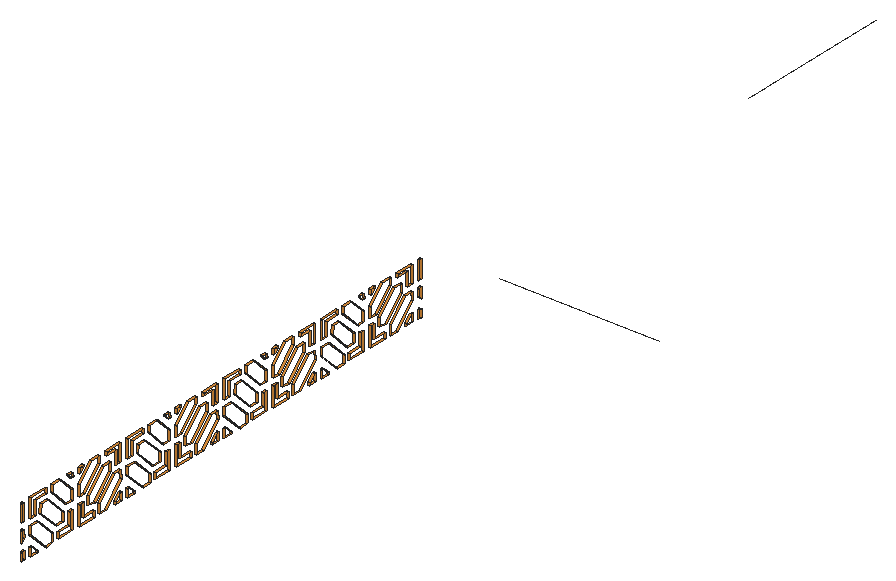
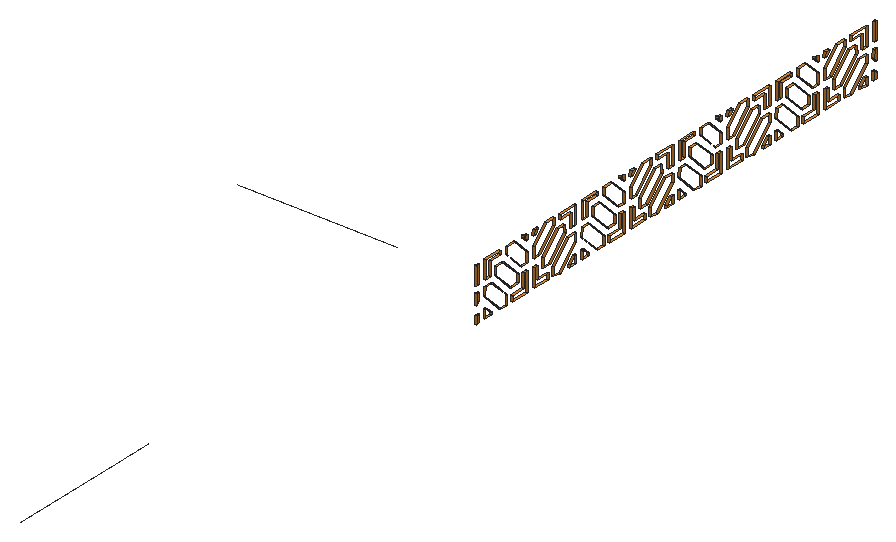
# SketchUp Ruby script. Lengths in inches.
U = 1.inch
M = Sketchup.active_model
def pt(a) = Geom::Point3d.new(a.map { |v| v * U })
def face(e, loops, mat)
  f = e.add_face(loops[0].map { |a| pt(a) })
  loops[1..].each { |l| e.add_face(l.map { |a| pt(a) }).erase! }
  f.material = f.back_material = mat if mat
  f
end
# faces: each face lists its corners as indices into pts; further lists are holes
def faces(e, pts, list, mat = nil) = list.each { |f| face(e, (f[0].is_a?(Array) ? f : [f]).map { |l| l.map { |i| pts[i] } }, mat) }
# xy, xz, yz: faces in a plane at the given z, y or x. An outline is a flat list of corners, or four numbers for a rectangle; further outlines are holes
def ring(l) = l.size == 4 ? [[l[0], l[1]], [l[2], l[1]], [l[2], l[3]], [l[0], l[3]]] : l.each_slice(2).to_a
def flat(e, list, mat, &to3) = list.each { |f| face(e, (f[0].is_a?(Array) ? f : [f]).map { |l| ring(l).map { |u, v| to3.(u, v) } }, mat) }
def xy(e, z, list, mat = nil) = flat(e, list, mat) { |x, y| [x, y, z] }
def xz(e, y, list, mat = nil) = flat(e, list, mat) { |x, z| [x, y, z] }
def yz(e, x, list, mat = nil) = flat(e, list, mat) { |y, z| [x, y, z] }
def lines(e, pts, list) = list.each { |a, b| e.add_line(pt(pts[a]), pt(pts[b])) }
# prism: a flat outline (further loops are holes) pulled along v
def prism(e, loops, v, mat = nil)
  f = face(e, loops, mat); d = Geom::Vector3d.new(v.map { |x| x * U })
  f.pushpull(f.normal.samedirection?(d) ? d.length : -d.length)
end
def box(e, o, s, mat = nil) = prism(e, [[o, [o[0] + s[0], o[1], o[2]], [o[0] + s[0], o[1] + s[1], o[2]], [o[0], o[1] + s[1], o[2]]]], [0, 0, s[2]], mat)
def at(x, y, z, deg = 0) = Geom::Transformation.translation(pt([x, y, z])) * Geom::Transformation.rotation(ORIGIN, Z_AXIS, deg.degrees)
def axes(o, x, y, z) = Geom::Transformation.new([*x, 0, *y, 0, *z, 0, *pt(o).to_a, 1])
def part(name) = M.definitions.add(name)
# library, detail: a bought-in or finely detailed component or shape, given as its bounding box
def library(name, o, s) = part(name).tap { |d| box(d.entities, o, s) }
def detail(e, o, s) = box(e.add_group.entities, o, s)
def put(e, d, t, mat = nil) = e.add_instance(d, t).tap { |i| i.material = mat if mat }
def group(e, t, mat = nil) = e.add_group.tap { |g| g.transformation = t; g.material = mat if mat }.entities
root = M.entities
M.materials.add("1056 AP 9903 Mellow Melon-N").color = [219, 142, 59]
xy(root,193.38,[[14.35,18.88,15.0625,21.91],[14.35,64.22,15.0625,67.26],[14.35,109.57,15.0625,112.6],[14.35,154.91,15.0625,157.94],[14.35,200.25,15.0625,201.3125]],"1056 AP 9903 Mellow Melon-N")
xy(root,193.61,[[14.35,14.79,15.0625,16.07],[14.35,41.65,15.0625,48.53],[14.35,51.11,15.0625,54.08],[14.35,58.41,15.0625,61.42],[14.35,87,15.0625,93.87],
  [14.35,96.45,15.0625,99.42],[14.35,103.75,15.0625,106.76],[14.35,132.34,15.0625,139.21],[14.35,141.79,15.0625,144.77],[14.35,149.1,15.0625,152.1],
  [14.35,177.68,15.0625,184.56],[14.35,187.14,15.0625,190.11],[14.35,194.44,15.0625,197.45]],"1056 AP 9903 Mellow Melon-N")
xy(root,193.8125,[[14.35,31.88,15.0625,38.38],[14.35,77.22,15.0625,83.72],[14.35,122.57,15.0625,129.07],[14.35,167.91,15.0625,174.41]],"1056 AP 9903 Mellow Melon-N")
xy(root,195.78,[[14.35,43.37,15.0625,48.53],[14.35,88.72,15.0625,93.87],[14.35,134.06,15.0625,139.21],[14.35,179.4,15.0625,184.56]],"1056 AP 9903 Mellow Melon-N")
xy(root,195.96,[[14.35,31.88,15.0625,37.08],[14.35,77.22,15.0625,82.42],[14.35,122.57,15.0625,127.77],[14.35,167.91,15.0625,173.11]],"1056 AP 9903 Mellow Melon-N")
xy(root,196.39,[[14.35,18.88,15.0625,19.75],[14.35,64.22,15.0625,65.1],[14.35,109.57,15.0625,110.44],[14.35,154.91,15.0625,155.79],[14.35,200.25,15.0625,201.13]],"1056 AP 9903 Mellow Melon-N")
xy(root,196.64,[[14.35,15.22,15.0625,16.07],[14.35,60.57,15.0625,61.42],[14.35,105.91,15.0625,106.76],[14.35,151.25,15.0625,152.1],[14.35,196.6,15.0625,197.45]],"1056 AP 9903 Mellow Melon-N")
xy(root,198.54,[[14.35,30.98,15.0625,34.05],[14.35,76.32,15.0625,79.39],[14.35,121.67,15.0625,124.73],[14.35,167.01,15.0625,170.08]],"1056 AP 9903 Mellow Melon-N")
xy(root,200.6875,[[14.35,37.08,15.0625,38.38],[14.35,82.42,15.0625,83.72],[14.35,127.77,15.0625,129.07],[14.35,173.11,15.0625,174.41]],"1056 AP 9903 Mellow Melon-N")
xy(root,200.98,[[14.35,41.65,15.0625,43.37],[14.35,87,15.0625,88.72],[14.35,132.34,15.0625,134.06],[14.35,177.68,15.0625,179.4]],"1056 AP 9903 Mellow Melon-N")
xy(root,203.58,[[14.35,41.65,15.0625,44.2],[14.35,87,15.0625,89.54],[14.35,132.34,15.0625,134.89],[14.35,177.68,15.0625,180.23]],"1056 AP 9903 Mellow Melon-N")
xy(root,203.69,[[14.35,18.88,15.0625,22.375],[14.35,35.75,15.0625,38.38],[14.35,64.22,15.0625,67.72],[14.35,81.09,15.0625,83.72],[14.35,109.57,15.0625,113.0625],
  [14.35,126.4375,15.0625,129.07],[14.35,154.91,15.0625,158.41],[14.35,171.78,15.0625,174.41],[14.35,200.25,15.0625,201.3125]],"1056 AP 9903 Mellow Melon-N")
xy(root,204.01,[[14.35,14.79,15.0625,15.64],[14.35,58.01,15.0625,60.99],[14.35,103.35,15.0625,106.33],[14.35,148.7,15.0625,151.67],[14.35,194.04,15.0625,197.02]],"1056 AP 9903 Mellow Melon-N")
xy(root,206.27,[[14.35,18.88,15.0625,21.05],[14.35,64.22,15.0625,66.39],[14.35,109.57,15.0625,111.73],[14.35,154.91,15.0625,157.08],[14.35,200.25,15.0625,201.3125]],"1056 AP 9903 Mellow Melon-N")
xy(root,206.61,[[14.35,14.79,15.0625,15.64],[14.35,58.84,15.0625,60.99],[14.35,104.18,15.0625,106.33],[14.35,149.53,15.0625,151.67],[14.35,194.87,15.0625,197.02]],"1056 AP 9903 Mellow Melon-N")
xy(root,208.78,[[14.35,52.85,15.0625,56.26],[14.35,98.2,15.0625,101.6],[14.35,143.54,15.0625,146.95],[14.35,188.88,15.0625,192.29]],"1056 AP 9903 Mellow Melon-N")
xy(root,208.85,[[14.35,24.08,15.0625,27.14],[14.35,69.42,15.0625,72.49],[14.35,114.77,15.0625,117.83],[14.35,160.11,15.0625,163.17]],"1056 AP 9903 Mellow Melon-N")
xy(root,211.38,[[14.35,41.65,15.0625,42.08],[14.35,87,15.0625,87.42],[14.35,132.34,15.0625,132.76],[14.35,177.68,15.0625,178.11]],"1056 AP 9903 Mellow Melon-N")
xy(root,211.43,[[14.35,21.05,15.0625,26.25],[14.35,37.94,15.0625,38.8125],[14.35,66.39,15.0625,71.59],[14.35,83.29,15.0625,84.16],[14.35,111.73,15.0625,116.93],
  [14.35,128.63,15.0625,129.5],[14.35,157.08,15.0625,162.28],[14.35,173.97,15.0625,174.84]],"1056 AP 9903 Mellow Melon-N")
xy(root,211.8125,[[14.35,54.11,15.0625,58.84],[14.35,99.46,15.0625,104.18],[14.35,144.8,15.0625,149.53],[14.35,190.14,15.0625,194.87]],"1056 AP 9903 Mellow Melon-N")
xy(root,213.11,[[14.35,14.79,15.0625,15.64],[14.35,47.26,15.0625,51.11],[14.35,54.11,15.0625,60.99],[14.35,92.61,15.0625,96.45],[14.35,99.46,15.0625,106.33],
  [14.35,137.95,15.0625,141.79],[14.35,144.8,15.0625,151.67],[14.35,183.29,15.0625,187.14],[14.35,190.14,15.0625,197.02]],"1056 AP 9903 Mellow Melon-N")
xy(root,213.15,[[14.35,18.88,15.0625,26.25],[14.35,28.85,15.0625,32.77],[14.35,36.65,15.0625,38.38],[14.35,64.22,15.0625,71.59],[14.35,74.19,15.0625,78.11],
  [14.35,81.99,15.0625,83.72],[14.35,109.57,15.0625,116.93],[14.35,119.53,15.0625,123.46],[14.35,127.33,15.0625,129.07],[14.35,154.91,15.0625,162.28],
  [14.35,164.88,15.0625,168.8],[14.35,172.68,15.0625,174.41],[14.35,200.25,15.0625,201.3125]],"1056 AP 9903 Mellow Melon-N")
xz(root,14.79,[[14.35,193.61,15.0625,196.21],[14.35,199.66,15.0625,204.01],[14.35,206.61,15.0625,213.11]],"1056 AP 9903 Mellow Melon-N")
xz(root,15.64,[[14.35,206.61,15.0625,213.11]],"1056 AP 9903 Mellow Melon-N")
xz(root,16.07,[[14.35,193.61,15.0625,196.64]],"1056 AP 9903 Mellow Melon-N")
xz(root,18.88,[[14.35,193.38,15.0625,196.39],[14.35,200.72,15.0625,203.69],[14.35,206.27,15.0625,213.15]],"1056 AP 9903 Mellow Melon-N")
xz(root,21.05,[[14.35,206.27,15.0625,211.43]],"1056 AP 9903 Mellow Melon-N")
xz(root,21.91,[[14.35,193.38,15.0625,194.23]],"1056 AP 9903 Mellow Melon-N")
xz(root,26.25,[[14.35,211.43,15.0625,213.15]],"1056 AP 9903 Mellow Melon-N")
xz(root,28.85,[[14.35,210.6,15.0625,213.15]],"1056 AP 9903 Mellow Melon-N")
xz(root,29.28,[[14.35,193.8125,15.0625,196.79]],"1056 AP 9903 Mellow Melon-N")
xz(root,31.88,[[14.35,193.8125,15.0625,195.96]],"1056 AP 9903 Mellow Melon-N")
xz(root,34.05,[[14.35,198.54,15.0625,201.95]],"1056 AP 9903 Mellow Melon-N")
xz(root,36.65,[[14.35,212.72,15.0625,213.15]],"1056 AP 9903 Mellow Melon-N")
xz(root,37.08,[[14.35,195.96,15.0625,200.6875]],"1056 AP 9903 Mellow Melon-N")
xz(root,38.38,[[14.35,193.8125,15.0625,200.6875],[14.35,203.69,15.0625,207.54]],"1056 AP 9903 Mellow Melon-N")
xz(root,41.65,[[14.35,193.61,15.0625,200.98],[14.35,203.58,15.0625,207.5],[14.35,211.38,15.0625,213.11]],"1056 AP 9903 Mellow Melon-N")
xz(root,43.37,[[14.35,195.78,15.0625,200.98],[14.35,212.67,15.0625,213.55]],"1056 AP 9903 Mellow Melon-N")
xz(root,45.95,[[14.35,198.8125,15.0625,201.875]],"1056 AP 9903 Mellow Melon-N")
xz(root,48.53,[[14.35,193.61,15.0625,195.78]],"1056 AP 9903 Mellow Melon-N")
xz(root,51.11,[[14.35,193.61,15.0625,197.11],[14.35,210.48,15.0625,213.11]],"1056 AP 9903 Mellow Melon-N")
xz(root,54.11,[[14.35,211.8125,15.0625,213.11]],"1056 AP 9903 Mellow Melon-N")
xz(root,56.26,[[14.35,205.71,15.0625,208.78]],"1056 AP 9903 Mellow Melon-N")
xz(root,58.41,[[14.35,193.61,15.0625,194.49]],"1056 AP 9903 Mellow Melon-N")
xz(root,58.84,[[14.35,206.61,15.0625,211.8125]],"1056 AP 9903 Mellow Melon-N")
xz(root,60.99,[[14.35,206.61,15.0625,213.11]],"1056 AP 9903 Mellow Melon-N")
xz(root,61.42,[[14.35,193.61,15.0625,196.64]],"1056 AP 9903 Mellow Melon-N")
xz(root,64.22,[[14.35,193.38,15.0625,196.39],[14.35,200.72,15.0625,203.69],[14.35,206.27,15.0625,213.15]],"1056 AP 9903 Mellow Melon-N")
xz(root,66.39,[[14.35,206.27,15.0625,211.43]],"1056 AP 9903 Mellow Melon-N")
xz(root,67.26,[[14.35,193.38,15.0625,194.23]],"1056 AP 9903 Mellow Melon-N")
xz(root,71.59,[[14.35,211.43,15.0625,213.15]],"1056 AP 9903 Mellow Melon-N")
xz(root,74.19,[[14.35,210.6,15.0625,213.15]],"1056 AP 9903 Mellow Melon-N")
xz(root,74.625,[[14.35,193.8125,15.0625,196.79]],"1056 AP 9903 Mellow Melon-N")
xz(root,77.22,[[14.35,193.8125,15.0625,195.96]],"1056 AP 9903 Mellow Melon-N")
xz(root,79.39,[[14.35,198.54,15.0625,201.95]],"1056 AP 9903 Mellow Melon-N")
xz(root,81.99,[[14.35,212.72,15.0625,213.15]],"1056 AP 9903 Mellow Melon-N")
xz(root,82.42,[[14.35,195.96,15.0625,200.6875]],"1056 AP 9903 Mellow Melon-N")
xz(root,83.72,[[14.35,193.8125,15.0625,200.6875],[14.35,203.69,15.0625,207.54]],"1056 AP 9903 Mellow Melon-N")
xz(root,87,[[14.35,193.61,15.0625,200.98],[14.35,203.58,15.0625,207.5],[14.35,211.38,15.0625,213.11]],"1056 AP 9903 Mellow Melon-N")
xz(root,88.72,[[14.35,195.78,15.0625,200.98],[14.35,212.67,15.0625,213.55]],"1056 AP 9903 Mellow Melon-N")
xz(root,91.29,[[14.35,198.8125,15.0625,201.875]],"1056 AP 9903 Mellow Melon-N")
xz(root,93.87,[[14.35,193.61,15.0625,195.78]],"1056 AP 9903 Mellow Melon-N")
xz(root,96.45,[[14.35,193.61,15.0625,197.11],[14.35,210.48,15.0625,213.11]],"1056 AP 9903 Mellow Melon-N")
xz(root,99.46,[[14.35,211.8125,15.0625,213.11]],"1056 AP 9903 Mellow Melon-N")
xz(root,101.6,[[14.35,205.71,15.0625,208.78]],"1056 AP 9903 Mellow Melon-N")
xz(root,103.75,[[14.35,193.61,15.0625,194.49]],"1056 AP 9903 Mellow Melon-N")
xz(root,104.18,[[14.35,206.61,15.0625,211.8125]],"1056 AP 9903 Mellow Melon-N")
xz(root,106.33,[[14.35,206.61,15.0625,213.11]],"1056 AP 9903 Mellow Melon-N")
xz(root,106.76,[[14.35,193.61,15.0625,196.64]],"1056 AP 9903 Mellow Melon-N")
xz(root,109.57,[[14.35,193.38,15.0625,196.39],[14.35,200.72,15.0625,203.69],[14.35,206.27,15.0625,213.15]],"1056 AP 9903 Mellow Melon-N")
xz(root,111.73,[[14.35,206.27,15.0625,211.43]],"1056 AP 9903 Mellow Melon-N")
xz(root,112.6,[[14.35,193.38,15.0625,194.23]],"1056 AP 9903 Mellow Melon-N")
xz(root,116.93,[[14.35,211.43,15.0625,213.15]],"1056 AP 9903 Mellow Melon-N")
xz(root,119.53,[[14.35,210.6,15.0625,213.15]],"1056 AP 9903 Mellow Melon-N")
xz(root,119.97,[[14.35,193.8125,15.0625,196.79]],"1056 AP 9903 Mellow Melon-N")
xz(root,122.57,[[14.35,193.8125,15.0625,195.96]],"1056 AP 9903 Mellow Melon-N")
xz(root,124.73,[[14.35,198.54,15.0625,201.95]],"1056 AP 9903 Mellow Melon-N")
xz(root,127.33,[[14.35,212.72,15.0625,213.15]],"1056 AP 9903 Mellow Melon-N")
xz(root,127.77,[[14.35,195.96,15.0625,200.6875]],"1056 AP 9903 Mellow Melon-N")
xz(root,129.07,[[14.35,193.8125,15.0625,200.6875],[14.35,203.69,15.0625,207.54]],"1056 AP 9903 Mellow Melon-N")
xz(root,132.34,[[14.35,193.61,15.0625,200.98],[14.35,203.58,15.0625,207.5],[14.35,211.38,15.0625,213.11]],"1056 AP 9903 Mellow Melon-N")
xz(root,134.06,[[14.35,195.78,15.0625,200.98],[14.35,212.67,15.0625,213.55]],"1056 AP 9903 Mellow Melon-N")
xz(root,136.64,[[14.35,198.8125,15.0625,201.875]],"1056 AP 9903 Mellow Melon-N")
xz(root,139.21,[[14.35,193.61,15.0625,195.78]],"1056 AP 9903 Mellow Melon-N")
xz(root,141.79,[[14.35,193.61,15.0625,197.11],[14.35,210.48,15.0625,213.11]],"1056 AP 9903 Mellow Melon-N")
xz(root,144.8,[[14.35,211.8125,15.0625,213.11]],"1056 AP 9903 Mellow Melon-N")
xz(root,146.95,[[14.35,205.71,15.0625,208.78]],"1056 AP 9903 Mellow Melon-N")
xz(root,149.1,[[14.35,193.61,15.0625,194.49]],"1056 AP 9903 Mellow Melon-N")
xz(root,149.53,[[14.35,206.61,15.0625,211.8125]],"1056 AP 9903 Mellow Melon-N")
xz(root,151.67,[[14.35,206.61,15.0625,213.11]],"1056 AP 9903 Mellow Melon-N")
xz(root,152.1,[[14.35,193.61,15.0625,196.64]],"1056 AP 9903 Mellow Melon-N")
xz(root,154.91,[[14.35,193.38,15.0625,196.39],[14.35,200.72,15.0625,203.69],[14.35,206.27,15.0625,213.15]],"1056 AP 9903 Mellow Melon-N")
xz(root,157.08,[[14.35,206.27,15.0625,211.43]],"1056 AP 9903 Mellow Melon-N")
xz(root,157.94,[[14.35,193.38,15.0625,194.23]],"1056 AP 9903 Mellow Melon-N")
xz(root,162.28,[[14.35,211.43,15.0625,213.15]],"1056 AP 9903 Mellow Melon-N")
xz(root,164.88,[[14.35,210.6,15.0625,213.15]],"1056 AP 9903 Mellow Melon-N")
xz(root,165.3125,[[14.35,193.8125,15.0625,196.79]],"1056 AP 9903 Mellow Melon-N")
xz(root,167.91,[[14.35,193.8125,15.0625,195.96]],"1056 AP 9903 Mellow Melon-N")
xz(root,170.08,[[14.35,198.54,15.0625,201.95]],"1056 AP 9903 Mellow Melon-N")
xz(root,172.68,[[14.35,212.72,15.0625,213.15]],"1056 AP 9903 Mellow Melon-N")
xz(root,173.11,[[14.35,195.96,15.0625,200.6875]],"1056 AP 9903 Mellow Melon-N")
xz(root,174.41,[[14.35,193.8125,15.0625,200.6875],[14.35,203.69,15.0625,207.54]],"1056 AP 9903 Mellow Melon-N")
xz(root,177.68,[[14.35,193.61,15.0625,200.98],[14.35,203.58,15.0625,207.5],[14.35,211.38,15.0625,213.11]],"1056 AP 9903 Mellow Melon-N")
xz(root,179.4,[[14.35,195.78,15.0625,200.98],[14.35,212.67,15.0625,213.55]],"1056 AP 9903 Mellow Melon-N")
xz(root,181.98,[[14.35,198.8125,15.0625,201.875]],"1056 AP 9903 Mellow Melon-N")
xz(root,184.56,[[14.35,193.61,15.0625,195.78]],"1056 AP 9903 Mellow Melon-N")
xz(root,187.14,[[14.35,193.61,15.0625,197.11],[14.35,210.48,15.0625,213.11]],"1056 AP 9903 Mellow Melon-N")
xz(root,190.14,[[14.35,211.8125,15.0625,213.11]],"1056 AP 9903 Mellow Melon-N")
xz(root,192.29,[[14.35,205.71,15.0625,208.78]],"1056 AP 9903 Mellow Melon-N")
xz(root,194.44,[[14.35,193.61,15.0625,194.49]],"1056 AP 9903 Mellow Melon-N")
xz(root,194.87,[[14.35,206.61,15.0625,211.8125]],"1056 AP 9903 Mellow Melon-N")
xz(root,197.02,[[14.35,206.61,15.0625,213.11]],"1056 AP 9903 Mellow Melon-N")
xz(root,197.45,[[14.35,193.61,15.0625,196.64]],"1056 AP 9903 Mellow Melon-N")
xz(root,200.25,[[14.35,193.38,15.0625,196.39],[14.35,200.72,15.0625,203.69],[14.35,206.27,15.0625,213.15]],"1056 AP 9903 Mellow Melon-N")
xz(root,201.3125,[[14.35,193.38,15.0625,196.21],[14.35,199.66,15.0625,203.69],[14.35,206.27,15.0625,213.15]],"1056 AP 9903 Mellow Melon-N")
p = [[15.0625,18.88,200.72],[15.0625,26.22,193.38],[14.35,26.22,193.38],[14.35,18.88,200.72],[15.0625,29.28,193.8125],[14.35,29.28,193.8125],
  [15.0625,64.22,200.72],[15.0625,71.5625,193.38],[14.35,71.5625,193.38],[14.35,64.22,200.72],[15.0625,74.625,193.8125],[14.35,74.625,193.8125],
  [15.0625,109.57,200.72],[15.0625,116.91,193.38],[14.35,116.91,193.38],[14.35,109.57,200.72],[15.0625,119.97,193.8125],[14.35,119.97,193.8125],
  [15.0625,154.91,200.72],[15.0625,162.25,193.38],[14.35,162.25,193.38],[14.35,154.91,200.72],[15.0625,165.3125,193.8125],[14.35,165.3125,193.8125],
  [15.0625,54.08,193.61],[15.0625,61.42,200.95],[14.35,61.42,200.95],[14.35,54.08,193.61],[15.0625,99.42,193.61],[15.0625,106.76,200.95],
  [14.35,106.76,200.95],[14.35,99.42,193.61],[15.0625,144.77,193.61],[15.0625,152.11,200.95],[14.35,152.11,200.95],[14.35,144.77,193.61],
  [15.0625,190.11,193.61],[15.0625,197.45,200.95],[14.35,197.45,200.95],[14.35,190.11,193.61],[15.0625,21.91,194.23],[15.0625,19.75,196.39],
  [14.35,19.75,196.39],[14.35,21.91,194.23],[15.0625,67.26,194.23],[15.0625,65.1,196.39],[14.35,65.1,196.39],[14.35,67.26,194.23],
  [15.0625,112.6,194.23],[15.0625,110.44,196.39],[14.35,110.44,196.39],[14.35,112.6,194.23],[15.0625,157.94,194.23],[15.0625,155.79,196.39],
  [14.35,155.79,196.39],[14.35,157.94,194.23],[15.0625,60.57,196.64],[15.0625,58.41,194.49],[14.35,58.41,194.49],[14.35,60.57,196.64],
  [15.0625,105.91,196.64],[15.0625,103.75,194.49],[14.35,103.75,194.49],[14.35,105.91,196.64],[15.0625,151.25,196.64],[15.0625,149.1,194.49],
  [14.35,149.1,194.49],[14.35,151.25,196.64],[15.0625,196.6,196.64],[15.0625,194.44,194.49],[14.35,194.44,194.49],[14.35,196.6,196.64],
  [15.0625,15.22,196.64],[15.0625,14.79,196.21],[14.35,14.79,196.21],[14.35,15.22,196.64],[15.0625,201.3125,196.21],[15.0625,201.13,196.39],
  [14.35,201.13,196.39],[14.35,201.3125,196.21],[15.0625,29.28,196.79],[15.0625,22.375,203.69],[14.35,22.375,203.69],[14.35,29.28,196.79],
  [15.0625,74.625,196.79],[15.0625,67.72,203.69],[14.35,67.72,203.69],[14.35,74.625,196.79],[15.0625,119.97,196.79],[15.0625,113.0625,203.69],
  [14.35,113.0625,203.69],[14.35,119.97,196.79],[15.0625,165.3125,196.79],[15.0625,158.41,203.69],[14.35,158.41,203.69],[14.35,165.3125,196.79],
  [15.0625,58.01,204.01],[15.0625,51.11,197.11],[14.35,51.11,197.11],[14.35,58.01,204.01],[15.0625,103.35,204.01],[15.0625,96.45,197.11],
  [14.35,96.45,197.11],[14.35,103.35,204.01],[15.0625,148.7,204.01],[15.0625,141.79,197.11],[14.35,141.79,197.11],[14.35,148.7,204.01],
  [15.0625,194.04,204.01],[15.0625,187.14,197.11],[14.35,187.14,197.11],[14.35,194.04,204.01],[15.0625,45.95,198.8125],[15.0625,48.93,198.38],
  [14.35,48.93,198.38],[14.35,45.95,198.8125],[15.0625,56.26,205.71],[14.35,56.26,205.71],[15.0625,91.29,198.8125],[15.0625,94.27,198.38],
  [14.35,94.27,198.38],[14.35,91.29,198.8125],[15.0625,101.6,205.71],[14.35,101.6,205.71],[15.0625,136.64,198.8125],[15.0625,139.62,198.38],
  [14.35,139.62,198.38],[14.35,136.64,198.8125],[15.0625,146.95,205.71],[14.35,146.95,205.71],[15.0625,181.98,198.8125],[15.0625,184.96,198.38],
  [14.35,184.96,198.38],[14.35,181.98,198.8125],[15.0625,192.29,205.71],[14.35,192.29,205.71],[15.0625,23.65,205.87],[15.0625,30.98,198.54],
  [14.35,30.98,198.54],[14.35,23.65,205.87],[15.0625,68.99,205.87],[15.0625,76.32,198.54],[14.35,76.32,198.54],[14.35,68.99,205.87],
  [15.0625,114.34,205.87],[15.0625,121.67,198.54],[14.35,121.67,198.54],[14.35,114.34,205.87],[15.0625,159.68,205.87],[15.0625,167.01,198.54],
  [14.35,167.01,198.54],[14.35,159.68,205.87],[15.0625,14.79,199.66],[15.0625,16.08,200.95],[14.35,16.08,200.95],[14.35,14.79,199.66],
  [15.0625,200.25,200.72],[15.0625,201.3125,199.66],[14.35,201.3125,199.66],[14.35,200.25,200.72],[15.0625,15.64,204.01],[14.35,15.64,204.01],
  [15.0625,60.99,204.01],[14.35,60.99,204.01],[15.0625,106.33,204.01],[14.35,106.33,204.01],[15.0625,151.67,204.01],[14.35,151.67,204.01],
  [15.0625,197.02,204.01],[14.35,197.02,204.01],[15.0625,34.05,201.95],[15.0625,27.14,208.85],[14.35,27.14,208.85],[14.35,34.05,201.95],
  [15.0625,52.85,208.78],[15.0625,45.95,201.875],[14.35,45.95,201.875],[14.35,52.85,208.78],[15.0625,79.39,201.95],[15.0625,72.49,208.85],
  [14.35,72.49,208.85],[14.35,79.39,201.95],[15.0625,98.2,208.78],[15.0625,91.29,201.875],[14.35,91.29,201.875],[14.35,98.2,208.78],
  [15.0625,124.73,201.95],[15.0625,117.83,208.85],[14.35,117.83,208.85],[14.35,124.73,201.95],[15.0625,143.54,208.78],[15.0625,136.64,201.875],
  [14.35,136.64,201.875],[14.35,143.54,208.78],[15.0625,170.08,201.95],[15.0625,163.17,208.85],[14.35,163.17,208.85],[14.35,170.08,201.95],
  [15.0625,188.88,208.78],[15.0625,181.98,201.875],[14.35,181.98,201.875],[14.35,188.88,208.78],[15.0625,44.2,203.58],[15.0625,51.11,210.48],
  [14.35,51.11,210.48],[14.35,44.2,203.58],[15.0625,89.54,203.58],[15.0625,96.45,210.48],[14.35,96.45,210.48],[14.35,89.54,203.58],
  [15.0625,134.89,203.58],[15.0625,141.79,210.48],[14.35,141.79,210.48],[14.35,134.89,203.58],[15.0625,180.23,203.58],[15.0625,187.14,210.48],
  [14.35,187.14,210.48],[14.35,180.23,203.58],[15.0625,28.85,210.6],[15.0625,35.75,203.69],[14.35,35.75,203.69],[14.35,28.85,210.6],
  [15.0625,74.19,210.6],[15.0625,81.09,203.69],[14.35,81.09,203.69],[14.35,74.19,210.6],[15.0625,119.53,210.6],[15.0625,126.4375,203.69],
  [14.35,126.4375,203.69],[14.35,119.53,210.6],[15.0625,164.88,210.6],[15.0625,171.78,203.69],[14.35,171.78,203.69],[14.35,164.88,210.6],
  [15.0625,24.08,208.85],[14.35,24.08,208.85],[15.0625,69.42,208.85],[14.35,69.42,208.85],[15.0625,114.77,208.85],[14.35,114.77,208.85],
  [15.0625,160.11,208.85],[14.35,160.11,208.85],[15.0625,38.38,207.54],[15.0625,32.77,213.15],[14.35,32.77,213.15],[14.35,38.38,207.54],
  [15.0625,47.26,213.11],[15.0625,41.65,207.5],[14.35,41.65,207.5],[14.35,47.26,213.11],[15.0625,83.72,207.54],[15.0625,78.11,213.15],
  [14.35,78.11,213.15],[14.35,83.72,207.54],[15.0625,92.61,213.11],[15.0625,87,207.5],[14.35,87,207.5],[14.35,92.61,213.11],
  [15.0625,129.07,207.54],[15.0625,123.46,213.15],[14.35,123.46,213.15],[14.35,129.07,207.54],[15.0625,137.95,213.11],[15.0625,132.34,207.5],
  [14.35,132.34,207.5],[14.35,137.95,213.11],[15.0625,174.41,207.54],[15.0625,168.8,213.15],[14.35,168.8,213.15],[14.35,174.41,207.54],
  [15.0625,183.29,213.11],[15.0625,177.68,207.5],[14.35,177.68,207.5],[14.35,183.29,213.11],[15.0625,36.65,212.72],[15.0625,37.94,211.43],
  [14.35,37.94,211.43],[14.35,36.65,212.72],[15.0625,38.8125,211.43],[15.0625,38.38,213.15],[14.35,38.38,213.15],[14.35,38.8125,211.43],
  [15.0625,42.08,211.38],[15.0625,43.37,212.67],[14.35,43.37,212.67],[14.35,42.08,211.38],[15.0625,81.99,212.72],[15.0625,83.29,211.43],
  [14.35,83.29,211.43],[14.35,81.99,212.72],[15.0625,84.16,211.43],[15.0625,83.72,213.15],[14.35,83.72,213.15],[14.35,84.16,211.43],
  [15.0625,87.42,211.38],[15.0625,88.72,212.67],[14.35,88.72,212.67],[14.35,87.42,211.38],[15.0625,127.33,212.72],[15.0625,128.63,211.43],
  [14.35,128.63,211.43],[14.35,127.33,212.72],[15.0625,129.5,211.43],[15.0625,129.07,213.15],[14.35,129.07,213.15],[14.35,129.5,211.43],
  [15.0625,132.76,211.38],[15.0625,134.06,212.67],[14.35,134.06,212.67],[14.35,132.76,211.38],[15.0625,172.68,212.72],[15.0625,173.97,211.43],
  [14.35,173.97,211.43],[14.35,172.68,212.72],[15.0625,174.84,211.43],[15.0625,174.41,213.15],[14.35,174.41,213.15],[14.35,174.84,211.43],
  [15.0625,178.11,211.38],[15.0625,179.4,212.67],[14.35,179.4,212.67],[14.35,178.11,211.38],[15.0625,43.37,213.55],[15.0625,41.65,213.11],
  [14.35,41.65,213.11],[14.35,43.37,213.55],[15.0625,88.72,213.55],[15.0625,87,213.11],[14.35,87,213.11],[14.35,88.72,213.55],
  [15.0625,134.06,213.55],[15.0625,132.34,213.11],[14.35,132.34,213.11],[14.35,134.06,213.55],[15.0625,179.4,213.55],[15.0625,177.68,213.11],
  [14.35,177.68,213.11],[14.35,179.4,213.55],[26.375,339.5625,210],[26.375,399.5625,210],[39.5625,206.8125,212.75],[99.5625,206.8125,212.75]]
faces(root,p,[[0,1,2,3],[1,4,5,2],[6,7,8,9],[7,10,11,8],[12,13,14,15],[13,16,17,14],[18,19,20,21],[19,22,23,20],
  [24,25,26,27],[28,29,30,31],[32,33,34,35],[36,37,38,39],[40,41,42,43],[44,45,46,47],[48,49,50,51],[52,53,54,55],
  [56,57,58,59],[60,61,62,63],[64,65,66,67],[68,69,70,71],[72,73,74,75],[76,77,78,79],[80,81,82,83],[84,85,86,87],
  [88,89,90,91],[92,93,94,95],[96,97,98,99],[100,101,102,103],[104,105,106,107],[108,109,110,111],[112,113,114,115],[113,116,117,114],
  [118,119,120,121],[119,122,123,120],[124,125,126,127],[125,128,129,126],[130,131,132,133],[131,134,135,132],[136,137,138,139],[140,141,142,143],
  [144,145,146,147],[148,149,150,151],[152,153,154,155],[156,157,158,159],[153,160,161,154],[25,162,163,26],[29,164,165,30],[33,166,167,34],
  [37,168,169,38],[170,171,172,173],[174,175,176,177],[178,179,180,181],[182,183,184,185],[186,187,188,189],[190,191,192,193],[194,195,196,197],
  [198,199,200,201],[202,203,204,205],[206,207,208,209],[210,211,212,213],[214,215,216,217],[218,219,220,221],[222,223,224,225],[226,227,228,229],
  [230,231,232,233],[234,136,139,235],[236,140,143,237],[238,144,147,239],[240,148,151,241],[242,243,244,245],[246,247,248,249],[250,251,252,253],
  [254,255,256,257],[258,259,260,261],[262,263,264,265],[266,267,268,269],[270,271,272,273],[274,275,276,277],[278,279,280,281],[282,283,284,285],
  [286,287,288,289],[290,291,292,293],[294,295,296,297],[298,299,300,301],[302,303,304,305],[306,307,308,309],[310,311,312,313],[314,315,316,317],
  [318,319,320,321],[322,323,324,325],[326,327,328,329],[330,331,332,333],[334,335,336,337]],"1056 AP 9903 Mellow Melon-N")
lines(root,p,[[338,339],[340,341]])
